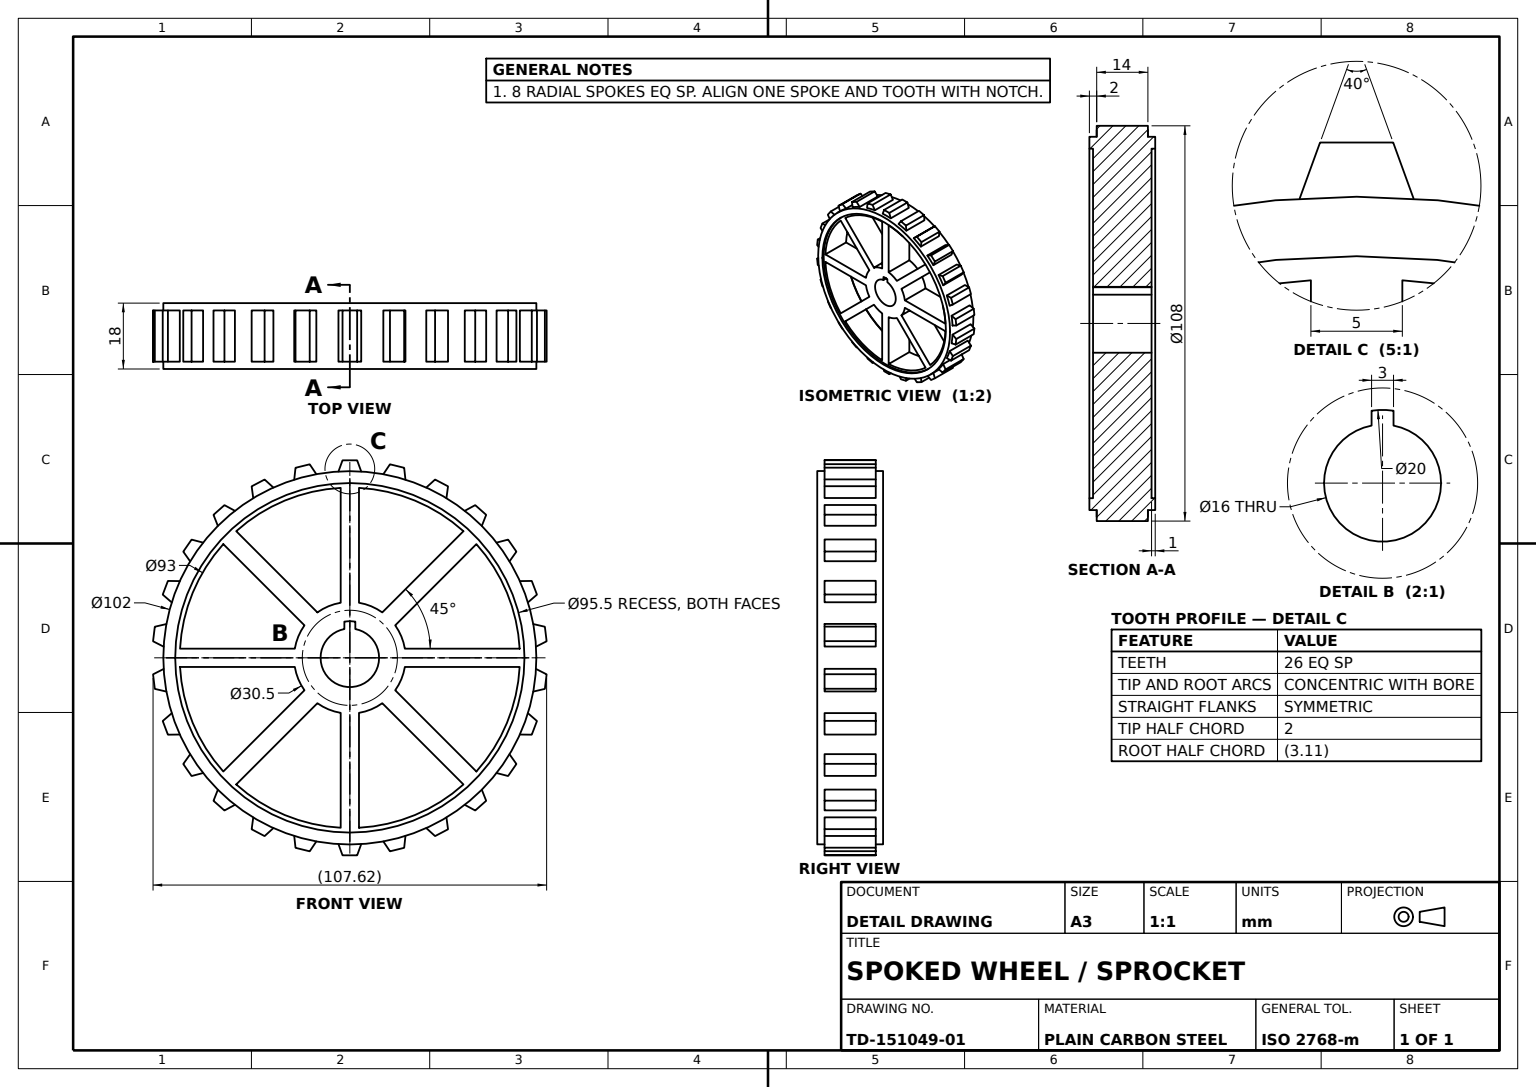
solid
v1 (51.165445,17.265493,7)
v2 (51.165445,17.265493,-7)
e1 v1 v2 LINE
v3 (48.700808,15.140385,7)
e2 v3 v1 LINE
v4 (48.700808,15.140385,-7)
e3 v3 v4 LINE
e4 v4 v2 LINE
face PLANE(AX(P(51.165445,17.265493,7),D(-0.653013985,0.757345849,0),D(-0.757345849,-0.653013985,0))) rev [-e1 -e2 e3 e4]
v5 (26.848745,46.852373,-7)
v6 (23.306921,48.711266,-7)
e5 v5 v6 CIRCLE(AX(P(0,0,-7),D(0,0,1),D(1,0,0)),54)
v7 (23.306921,48.711266,7)
e6 v7 v6 LINE
v8 (26.848745,46.852373,7)
e7 v8 v7 CIRCLE(AX(P(0,0,7),D(0,0,1),D(1,0,0)),54)
e8 v8 v5 LINE
face CYL(AX(P(0,0,7),D(0,0,-1),D(-1,0,0)),54) [e5 -e6 -e7 e8]
v9 (-34.287034,-41.718094,7)
v10 (-31.426051,-40.167192,7)
e9 v9 v10 LINE
v11 (-36.086337,-36.038539,7)
e10 v11 v10 CIRCLE(AX(P(0,0,7),D(0,0,1),D(1,0,0)),51)
v12 (-37.281077,-39.065603,7)
e11 v11 v12 LINE
e12 v12 v9 CIRCLE(AX(P(0,0,7),D(0,0,1),D(1,0,0)),54)
face PLANE(AX(P(0,0,7),D(0,0,1),D(1,0,0))) [e9 -e10 e11 e12]
v13 (53.810573,-4.519097,7)
v14 (50.908983,-3.045567,7)
e13 v13 v14 LINE
v15 (53.810573,-4.519097,-7)
e14 v13 v15 LINE
v16 (50.908983,-3.045567,-7)
e15 v15 v16 LINE
e16 v14 v16 LINE
face PLANE(AX(P(53.810573,-4.519097,7),D(-0.45279386,-0.891615231,0),D(0.891615231,-0.45279386,0))) rev [-e13 e14 e15 -e16]
v17 (-31.065143,34.600677,8)
v18 (-31.065143,34.600677,-8)
e17 v17 v18 LINE
v19 (-2.5,46.432747,-8)
e18 v18 v19 CIRCLE(AX(P(0,0,-8),D(0,0,-1),D(-1,0,0)),46.5)
v20 (-2.5,46.432747,8)
e19 v20 v19 LINE
e20 v20 v17 CIRCLE(AX(P(0,0,8),D(0,0,1),D(1,0,0)),46.5)
face CYL(AX(P(0,0,9),D(0,0,-1),D(-1,0,0)),46.5) rev [e17 e18 -e19 e20]
v21 (31.065143,34.600677,8)
v22 (2.5,46.432747,8)
e21 v21 v22 CIRCLE(AX(P(0,0,8),D(0,0,1),D(1,0,0)),46.5)
v23 (2.5,46.432747,-8)
e22 v22 v23 LINE
v24 (31.065143,34.600677,-8)
e23 v23 v24 CIRCLE(AX(P(0,0,-8),D(0,0,-1),D(-1,0,0)),46.5)
e24 v21 v24 LINE
face CYL(AX(P(0,0,9),D(0,0,-1),D(-1,0,0)),46.5) rev [e21 e22 e23 -e24]
v25 (51.165445,-17.265493,7)
v26 (48.700808,-15.140385,7)
e25 v25 v26 LINE
v27 (51.165445,-17.265493,-7)
e26 v25 v27 LINE
v28 (48.700808,-15.140385,-7)
e27 v27 v28 LINE
e28 v26 v28 LINE
face PLANE(AX(P(51.165445,-17.265493,7),D(-0.653013985,-0.757345849,0),D(0.757345849,-0.653013985,0))) rev [-e25 e26 e27 -e28]
v29 (-3.113039,-50.904901,-7)
v30 (-2,-53.96295,-7)
e29 v29 v30 LINE
v31 (-2,-53.96295,7)
e30 v31 v30 LINE
v32 (-3.113039,-50.904901,7)
e31 v32 v31 LINE
e32 v32 v29 LINE
face PLANE(AX(P(-2,-53.96295,7),D(0.939692621,0.342020143,0),D(-0.342020143,0.939692621,0))) rev [e29 -e30 -e31 e32]
v33 (-26.848745,-46.852373,7)
v34 (-26.848745,-46.852373,-7)
e33 v33 v34 LINE
v35 (-26.413146,-43.62735,7)
e34 v35 v33 LINE
v36 (-26.413146,-43.62735,-7)
e35 v35 v36 LINE
e36 v36 v34 LINE
face PLANE(AX(P(-26.848745,-46.852373,7),D(0.991001179,-0.133853139,0),D(0.133853139,0.991001179,0))) rev [-e33 -e34 e35 e36]
v37 (46.493011,20.961869,7)
e37 v3 v37 CIRCLE(AX(P(0,0,7),D(0,0,1),D(1,0,0)),51)
v38 (49.747025,21.005558,7)
e38 v1 v38 CIRCLE(AX(P(0,0,7),D(0,0,1),D(1,0,0)),54)
e39 v38 v37 LINE
face PLANE(AX(P(0,0,7),D(0,0,1),D(1,0,0))) [-e37 e2 e38 e39]
v39 (-20.900228,46.520753,-7)
v40 (-23.306921,48.711266,-7)
e40 v39 v40 LINE
v41 (-26.413146,43.62735,-7)
e41 v39 v41 CIRCLE(AX(P(0,0,-7),D(0,0,1),D(1,0,0)),51)
v42 (-26.848745,46.852373,-7)
e42 v42 v41 LINE
e43 v40 v42 CIRCLE(AX(P(0,0,-7),D(0,0,1),D(1,0,0)),54)
face PLANE(AX(P(0,0,-7),D(0,0,1),D(1,0,0))) rev [-e40 e41 -e42 -e43]
v43 (8.869726,12.40526,8)
e44 v43 v21 LINE
v44 (2.5,15.043686,8)
e45 v44 v43 CIRCLE(AX(P(0,0,8),D(0,0,-1),D(1,0,0)),15.25)
e46 v22 v44 LINE
v45 (-34.600677,31.065143,8)
v46 (-46.432747,2.5,8)
e47 v45 v46 CIRCLE(AX(P(0,0,8),D(0,0,1),D(1,0,0)),46.5)
v47 (-12.40526,8.869726,8)
e48 v47 v45 LINE
v48 (-15.043686,2.5,8)
e49 v48 v47 CIRCLE(AX(P(0,0,8),D(0,0,-1),D(1,0,0)),15.25)
e50 v46 v48 LINE
v49 (-8.869726,-12.40526,8)
v50 (-31.065143,-34.600677,8)
e51 v49 v50 LINE
v51 (-2.5,-15.043686,8)
e52 v51 v49 CIRCLE(AX(P(0,0,8),D(0,0,-1),D(1,0,0)),15.25)
v52 (-2.5,-46.432747,8)
e53 v52 v51 LINE
e54 v50 v52 CIRCLE(AX(P(0,0,8),D(0,0,1),D(1,0,0)),46.5)
v53 (-2.5,15.043686,8)
e55 v53 v20 LINE
v54 (-8.869726,12.40526,8)
e56 v54 v53 CIRCLE(AX(P(0,0,8),D(0,0,-1),D(1,0,0)),15.25)
e57 v17 v54 LINE
v55 (2.5,-15.043686,8)
v56 (2.5,-46.432747,8)
e58 v55 v56 LINE
v57 (8.869726,-12.40526,8)
e59 v57 v55 CIRCLE(AX(P(0,0,8),D(0,0,-1),D(1,0,0)),15.25)
v58 (31.065143,-34.600677,8)
e60 v58 v57 LINE
e61 v56 v58 CIRCLE(AX(P(0,0,8),D(0,0,1),D(1,0,0)),46.5)
v59 (-34.600677,-31.065143,8)
v60 (-12.40526,-8.869726,8)
e62 v59 v60 LINE
v61 (-46.432747,-2.5,8)
e63 v61 v59 CIRCLE(AX(P(0,0,8),D(0,0,1),D(1,0,0)),46.5)
v62 (-15.043686,-2.5,8)
e64 v62 v61 LINE
e65 v60 v62 CIRCLE(AX(P(0,0,8),D(0,0,-1),D(1,0,0)),15.25)
v63 (-47.75,0,8)
v64 (47.75,0,8)
e66 v63 v64 CIRCLE(AX(P(0,0,8),D(0,0,1),D(1,0,0)),47.75)
e67 v64 v63 CIRCLE(AX(P(0,0,8),D(0,0,1),D(1,0,0)),47.75)
v65 (1.5,9.88686,8)
v66 (1.5,7.858117,8)
e68 v65 v66 LINE
v67 (8,0,8)
e69 v67 v66 CIRCLE(AX(P(0,0,8),D(0,0,1),D(1,0,0)),8)
v68 (-8,0,8)
e70 v68 v67 CIRCLE(AX(P(0,0,8),D(0,0,1),D(1,0,0)),8)
v69 (-1.5,7.858117,8)
e71 v69 v68 CIRCLE(AX(P(0,0,8),D(0,0,1),D(1,0,0)),8)
v70 (-1.5,9.88686,8)
e72 v69 v70 LINE
e73 v70 v65 CIRCLE(AX(P(0,0,8),D(0,0,-1),D(1,0,0)),10)
v71 (15.043686,-2.5,8)
v72 (12.40526,-8.869726,8)
e74 v71 v72 CIRCLE(AX(P(0,0,8),D(0,0,-1),D(1,0,0)),15.25)
v73 (46.432747,-2.5,8)
e75 v73 v71 LINE
v74 (34.600677,-31.065143,8)
e76 v74 v73 CIRCLE(AX(P(0,0,8),D(0,0,1),D(1,0,0)),46.5)
e77 v72 v74 LINE
v75 (15.043686,2.5,8)
v76 (46.432747,2.5,8)
e78 v75 v76 LINE
v77 (12.40526,8.869726,8)
e79 v77 v75 CIRCLE(AX(P(0,0,8),D(0,0,-1),D(1,0,0)),15.25)
v78 (34.600677,31.065143,8)
e80 v78 v77 LINE
e81 v76 v78 CIRCLE(AX(P(0,0,8),D(0,0,1),D(1,0,0)),46.5)
face PLANE(AX(P(0,0,8),D(0,0,1),D(1,0,0))) [-e44 -e45 -e46 -e21] [-e47 -e48 -e49 -e50] [-e51 -e52 -e53 -e54] [-e20 -e55 -e56 -e57] [-e58 -e59 -e60 -e61] [-e62 -e63 -e64 -e65] [e66 e67] [e68 -e69 -e70 -e71 e72 e73] [-e74 -e75 -e76 -e77] [-e78 -e79 -e80 -e81]
v79 (9.159761,-50.170696,-7)
v80 (10.972296,-52.873516,-7)
e82 v79 v80 LINE
v81 (10.972296,-52.873516,7)
e83 v81 v80 LINE
v82 (9.159761,-50.170696,7)
e84 v82 v81 LINE
e85 v82 v79 LINE
face PLANE(AX(P(10.972296,-52.873516,7),D(0.830536083,0.556964823,0),D(-0.556964823,0.830536083,0))) rev [e82 -e83 -e84 e85]
v83 (15.043686,-2.5,-8)
e86 v71 v83 LINE
v84 (46.432747,-2.5,-8)
e87 v83 v84 LINE
e88 v73 v84 LINE
face PLANE(AX(P(46.432747,-2.5,9),D(0,-1,0),D(1,0,0))) [e86 e87 -e88 e75]
v85 (-34.600677,31.065143,-8)
e89 v45 v85 LINE
v86 (-12.40526,8.869726,-8)
e90 v85 v86 LINE
e91 v47 v86 LINE
face PLANE(AX(P(-12.40526,8.869726,9),D(-0.707106781,-0.707106781,0),D(0.707106781,-0.707106781,0))) [e89 e90 -e91 e48]
v87 (-48.700808,-15.140385,-7)
v88 (-51.165445,-17.265493,-7)
e92 v87 v88 LINE
v89 (-51.165445,-17.265493,7)
e93 v89 v88 LINE
v90 (-48.700808,-15.140385,7)
e94 v90 v89 LINE
e95 v90 v87 LINE
face PLANE(AX(P(-51.165445,-17.265493,7),D(0.653013985,-0.757345849,0),D(0.757345849,0.653013985,0))) rev [e92 -e93 -e94 e95]
v91 (50.158512,-9.226249,7)
v92 (53.328426,-8.489933,7)
e96 v91 v92 LINE
v93 (50.158512,-9.226249,-7)
e97 v91 v93 LINE
v94 (53.328426,-8.489933,-7)
e98 v93 v94 LINE
e99 v92 v94 LINE
face PLANE(AX(P(53.328426,-8.489933,7),D(-0.226259002,0.974067176,0),D(-0.974067176,-0.226259002,0))) rev [-e96 e97 e98 -e99]
v95 (14.856063,51.916254,-7)
v96 (10.972296,52.873516,-7)
e100 v95 v96 CIRCLE(AX(P(0,0,-7),D(0,0,1),D(1,0,0)),54)
v97 (10.972296,52.873516,7)
e101 v97 v96 LINE
v98 (14.856063,51.916254,7)
e102 v98 v97 CIRCLE(AX(P(0,0,7),D(0,0,1),D(1,0,0)),54)
e103 v98 v95 LINE
face CYL(AX(P(0,0,7),D(0,0,-1),D(-1,0,0)),54) [e100 -e101 -e102 e103]
v99 (34.287034,-41.718094,7)
v100 (34.287034,-41.718094,-7)
e104 v99 v100 LINE
v101 (37.281077,-39.065603,-7)
e105 v100 v101 CIRCLE(AX(P(0,0,-7),D(0,0,1),D(1,0,0)),54)
v102 (37.281077,-39.065603,7)
e106 v102 v101 LINE
e107 v99 v102 CIRCLE(AX(P(0,0,7),D(0,0,1),D(1,0,0)),54)
face CYL(AX(P(0,0,7),D(0,0,-1),D(-1,0,0)),54) [e104 e105 -e106 -e107]
v103 (-53.328426,8.489933,-7)
v104 (-53.810573,4.519097,-7)
e108 v103 v104 CIRCLE(AX(P(0,0,-7),D(0,0,1),D(1,0,0)),54)
v105 (-53.810573,4.519097,7)
e109 v105 v104 LINE
v106 (-53.328426,8.489933,7)
e110 v106 v105 CIRCLE(AX(P(0,0,7),D(0,0,1),D(1,0,0)),54)
e111 v106 v103 LINE
face CYL(AX(P(0,0,7),D(0,0,-1),D(-1,0,0)),54) [e108 -e109 -e110 e111]
v107 (20.900228,-46.520753,-7)
v108 (23.306921,-48.711266,-7)
e112 v107 v108 LINE
v109 (23.306921,-48.711266,7)
e113 v109 v108 LINE
v110 (20.900228,-46.520753,7)
e114 v110 v109 LINE
e115 v110 v107 LINE
face PLANE(AX(P(23.306921,-48.711266,7),D(0.673111807,0.739540732,0),D(-0.739540732,0.673111807,0))) rev [e112 -e113 -e114 e115]
v111 (50.908983,3.045567,7)
v112 (50.908983,3.045567,-7)
e116 v111 v112 LINE
v113 (53.810573,4.519097,-7)
e117 v112 v113 LINE
v114 (53.810573,4.519097,7)
e118 v114 v113 LINE
e119 v111 v114 LINE
face PLANE(AX(P(53.810573,4.519097,7),D(-0.45279386,0.891615231,0),D(-0.891615231,-0.45279386,0))) rev [e116 e117 -e118 -e119]
v115 (-37.281077,39.065603,7)
v116 (-36.086337,36.038539,7)
e120 v115 v116 LINE
v117 (-37.281077,39.065603,-7)
e121 v115 v117 LINE
v118 (-36.086337,36.038539,-7)
e122 v117 v118 LINE
e123 v116 v118 LINE
face PLANE(AX(P(-37.281077,39.065603,7),D(0.930171333,0.367125715,0),D(-0.367125715,0.930171333,0))) rev [-e120 e121 e122 -e123]
v119 (-46.432747,-2.5,-8)
e124 v61 v119 LINE
v120 (-15.043686,-2.5,-8)
e125 v119 v120 LINE
e126 v62 v120 LINE
face PLANE(AX(P(-15.043686,-2.5,9),D(0,-1,0),D(1,0,0))) [e124 e125 -e126 e64]
v121 (31.426051,40.167192,7)
v122 (31.426051,40.167192,-7)
e127 v121 v122 LINE
v123 (34.287034,41.718094,7)
e128 v123 v121 LINE
v124 (34.287034,41.718094,-7)
e129 v123 v124 LINE
e130 v124 v122 LINE
face PLANE(AX(P(34.287034,41.718094,7),D(0.47656872,-0.879137222,0),D(0.879137222,0.47656872,0))) rev [-e127 -e128 e129 e130]
v125 (-34.287034,41.718094,7)
e131 v125 v115 CIRCLE(AX(P(0,0,7),D(0,0,1),D(1,0,0)),54)
v126 (-31.426051,40.167192,7)
e132 v126 v116 CIRCLE(AX(P(0,0,7),D(0,0,1),D(1,0,0)),51)
e133 v126 v125 LINE
face PLANE(AX(P(0,0,7),D(0,0,1),D(1,0,0))) [e131 e120 -e132 e133]
v127 (-15.043686,2.5,-8)
v128 (-46.432747,2.5,-8)
e134 v127 v128 LINE
e135 v46 v128 LINE
e136 v48 v127 LINE
face PLANE(AX(P(-46.432747,2.5,9),D(0,1,0),D(-1,0,0))) [e134 -e135 e50 e136]
v129 (-36.086337,-36.038539,-7)
v130 (-31.426051,-40.167192,-7)
e137 v129 v130 CIRCLE(AX(P(0,0,-7),D(0,0,1),D(1,0,0)),51)
v131 (-34.287034,-41.718094,-7)
e138 v131 v130 LINE
v132 (-37.281077,-39.065603,-7)
e139 v132 v131 CIRCLE(AX(P(0,0,-7),D(0,0,1),D(1,0,0)),54)
e140 v129 v132 LINE
face PLANE(AX(P(0,0,-7),D(0,0,1),D(1,0,0))) rev [e137 -e138 -e139 -e140]
v133 (-49.747025,-21.005558,7)
v134 (-49.747025,-21.005558,-7)
e141 v133 v134 LINE
v135 (-46.493011,-20.961869,-7)
e142 v134 v135 LINE
v136 (-46.493011,-20.961869,7)
e143 v136 v135 LINE
e144 v133 v136 LINE
face PLANE(AX(P(-49.747025,-21.005558,7),D(-0.013425206,0.999909878,0),D(-0.999909878,-0.013425206,0))) rev [e141 e142 -e143 -e144]
v137 (-14.856063,51.916254,-7)
v138 (-15.20492,48.680699,-7)
e145 v137 v138 LINE
v139 (-10.972296,52.873516,-7)
e146 v139 v137 CIRCLE(AX(P(0,0,-7),D(0,0,1),D(1,0,0)),54)
v140 (-9.159761,50.170696,-7)
e147 v140 v139 LINE
e148 v140 v138 CIRCLE(AX(P(0,0,-7),D(0,0,1),D(1,0,0)),51)
face PLANE(AX(P(0,0,-7),D(0,0,1),D(1,0,0))) rev [-e145 -e146 -e147 e148]
e149 v89 v133 CIRCLE(AX(P(0,0,7),D(0,0,1),D(1,0,0)),54)
e150 v90 v136 CIRCLE(AX(P(0,0,7),D(0,0,1),D(1,0,0)),51)
face PLANE(AX(P(0,0,7),D(0,0,1),D(1,0,0))) [e94 e149 e144 -e150]
v141 (-49.747025,21.005558,-7)
v142 (-51.165445,17.265493,-7)
e151 v141 v142 CIRCLE(AX(P(0,0,-7),D(0,0,1),D(1,0,0)),54)
v143 (-51.165445,17.265493,7)
e152 v143 v142 LINE
v144 (-49.747025,21.005558,7)
e153 v144 v143 CIRCLE(AX(P(0,0,7),D(0,0,1),D(1,0,0)),54)
e154 v144 v141 LINE
face CYL(AX(P(0,0,7),D(0,0,-1),D(-1,0,0)),54) [e151 -e152 -e153 e154]
v145 (15.20492,-48.680699,7)
v146 (15.20492,-48.680699,-7)
e155 v145 v146 LINE
v147 (14.856063,-51.916254,7)
e156 v147 v145 LINE
v148 (14.856063,-51.916254,-7)
e157 v147 v148 LINE
e158 v148 v146 LINE
face PLANE(AX(P(14.856063,-51.916254,7),D(-0.994237639,0.107198496,0),D(-0.107198496,-0.994237639,0))) rev [-e155 -e156 e157 e158]
v149 (15.043686,2.5,-8)
e159 v75 v149 LINE
v150 (12.40526,8.869726,-8)
e160 v149 v150 CIRCLE(AX(P(0,0,-8),D(0,0,1),D(-1,0,0)),15.25)
e161 v77 v150 LINE
face CYL(AX(P(0,0,9),D(0,0,-1),D(-1,0,0)),15.25) [e159 e160 -e161 e79]
v151 (43.274508,32.300417,-7)
v152 (40.125505,31.479261,-7)
e162 v151 v152 LINE
v153 (40.125505,31.479261,7)
e163 v153 v152 LINE
v154 (43.274508,32.300417,7)
e164 v154 v153 LINE
e165 v154 v151 LINE
face PLANE(AX(P(43.274508,32.300417,7),D(0.252329191,-0.967641452,0),D(0.967641452,0.252329191,0))) rev [e162 -e163 -e164 e165]
v155 (-2.5,-46.432747,-8)
v156 (-31.065143,-34.600677,-8)
e166 v155 v156 CIRCLE(AX(P(0,0,-8),D(0,0,-1),D(-1,0,0)),46.5)
e167 v50 v156 LINE
e168 v52 v155 LINE
face CYL(AX(P(0,0,9),D(0,0,-1),D(-1,0,0)),46.5) rev [e166 -e167 e54 e168]
e169 v128 v85 CIRCLE(AX(P(0,0,-8),D(0,0,-1),D(-1,0,0)),46.5)
face CYL(AX(P(0,0,9),D(0,0,-1),D(-1,0,0)),46.5) rev [e169 -e89 e47 e135]
v157 (26.413146,43.62735,7)
e170 v157 v8 LINE
v158 (26.413146,43.62735,-7)
e171 v157 v158 LINE
e172 v158 v5 LINE
face PLANE(AX(P(26.848745,46.852373,7),D(-0.991001179,0.133853139,0),D(-0.133853139,-0.991001179,0))) rev [-e170 e171 e172 -e8]
v159 (-8.869726,-12.40526,-8)
e173 v156 v159 LINE
e174 v49 v159 LINE
face PLANE(AX(P(-8.869726,-12.40526,9),D(0.707106781,-0.707106781,0),D(0.707106781,0.707106781,0))) [e167 e173 -e174 e51]
v160 (46.432747,2.5,-8)
e175 v76 v160 LINE
e176 v160 v149 LINE
face PLANE(AX(P(15.043686,2.5,9),D(0,1,0),D(-1,0,0))) [-e159 e78 e175 e176]
v161 (2,53.96295,-7)
v162 (-2,53.96295,-7)
e177 v161 v162 CIRCLE(AX(P(0,0,-7),D(0,0,1),D(1,0,0)),54)
v163 (-2,53.96295,7)
e178 v163 v162 LINE
v164 (2,53.96295,7)
e179 v164 v163 CIRCLE(AX(P(0,0,7),D(0,0,1),D(1,0,0)),54)
e180 v164 v161 LINE
face CYL(AX(P(0,0,7),D(0,0,-1),D(-1,0,0)),54) [e177 -e178 -e179 e180]
v165 (31.065143,-34.600677,-8)
v166 (2.5,-46.432747,-8)
e181 v165 v166 CIRCLE(AX(P(0,0,-8),D(0,0,-1),D(-1,0,0)),46.5)
e182 v56 v166 LINE
e183 v58 v165 LINE
face CYL(AX(P(0,0,9),D(0,0,-1),D(-1,0,0)),46.5) rev [e181 -e182 e61 e183]
v167 (46.493011,20.961869,-7)
e184 v37 v167 LINE
v168 (49.747025,21.005558,-7)
e185 v38 v168 LINE
e186 v168 v167 LINE
face PLANE(AX(P(49.747025,21.005558,7),D(0.013425206,-0.999909878,0),D(0.999909878,0.013425206,0))) rev [-e184 -e39 e185 e186]
v169 (-34.287034,41.718094,-7)
e187 v125 v169 LINE
e188 v169 v117 CIRCLE(AX(P(0,0,-7),D(0,0,1),D(1,0,0)),54)
face CYL(AX(P(0,0,7),D(0,0,-1),D(-1,0,0)),54) [-e121 -e131 e187 e188]
e189 v92 v13 CIRCLE(AX(P(0,0,7),D(0,0,1),D(1,0,0)),54)
e190 v91 v14 CIRCLE(AX(P(0,0,7),D(0,0,1),D(1,0,0)),51)
face PLANE(AX(P(0,0,7),D(0,0,1),D(1,0,0))) [e96 e189 e13 -e190]
v170 (-40.125505,31.479261,7)
v171 (-43.274508,32.300417,7)
e191 v170 v171 LINE
v172 (-40.125505,31.479261,-7)
e192 v170 v172 LINE
v173 (-43.274508,32.300417,-7)
e193 v172 v173 LINE
e194 v171 v173 LINE
face PLANE(AX(P(-43.274508,32.300417,7),D(-0.252329191,-0.967641452,0),D(0.967641452,-0.252329191,0))) rev [-e191 e192 e193 -e194]
v174 (-12.40526,-8.869726,-8)
e195 v60 v174 LINE
v175 (-34.600677,-31.065143,-8)
e196 v174 v175 LINE
e197 v59 v175 LINE
face PLANE(AX(P(-34.600677,-31.065143,9),D(-0.707106781,0.707106781,0),D(-0.707106781,-0.707106781,0))) [e195 e196 -e197 e62]
v176 (49.747025,-21.005558,7)
e198 v176 v25 CIRCLE(AX(P(0,0,7),D(0,0,1),D(1,0,0)),54)
v177 (49.747025,-21.005558,-7)
e199 v176 v177 LINE
e200 v177 v27 CIRCLE(AX(P(0,0,-7),D(0,0,1),D(1,0,0)),54)
face CYL(AX(P(0,0,7),D(0,0,-1),D(-1,0,0)),54) [-e198 e199 e200 -e26]
v178 (-2.5,15.043686,-8)
e201 v53 v178 LINE
v179 (-8.869726,12.40526,-8)
e202 v178 v179 CIRCLE(AX(P(0,0,-8),D(0,0,1),D(-1,0,0)),15.25)
e203 v54 v179 LINE
face CYL(AX(P(0,0,9),D(0,0,-1),D(-1,0,0)),15.25) [e201 e202 -e203 e56]
v180 (-45.546767,29.008482,7)
v181 (-45.546767,29.008482,-7)
e204 v180 v181 LINE
e205 v171 v180 CIRCLE(AX(P(0,0,7),D(0,0,1),D(1,0,0)),54)
e206 v173 v181 CIRCLE(AX(P(0,0,-7),D(0,0,1),D(1,0,0)),54)
face CYL(AX(P(0,0,7),D(0,0,-1),D(-1,0,0)),54) [-e204 -e205 e194 e206]
v182 (-50.908983,3.045567,7)
v183 (-50.908983,3.045567,-7)
e207 v182 v183 LINE
e208 v105 v182 LINE
e209 v104 v183 LINE
face PLANE(AX(P(-53.810573,4.519097,7),D(0.45279386,0.891615231,0),D(-0.891615231,0.45279386,0))) rev [-e207 -e208 e109 e209]
v184 (-1.5,9.88686,-8)
e210 v184 v70 LINE
v185 (1.5,9.88686,-8)
e211 v185 v184 CIRCLE(AX(P(0,0,-8),D(0,0,1),D(-1,0,0)),10)
e212 v185 v65 LINE
face CYL(AX(P(0,0,-9),D(0,0,1),D(1,0,0)),10) rev [-e73 -e210 -e211 e212]
v186 (-14.856063,-51.916254,7)
v187 (-14.856063,-51.916254,-7)
e213 v186 v187 LINE
v188 (-15.20492,-48.680699,7)
e214 v188 v186 LINE
v189 (-15.20492,-48.680699,-7)
e215 v188 v189 LINE
e216 v189 v187 LINE
face PLANE(AX(P(-14.856063,-51.916254,7),D(0.994237639,0.107198496,0),D(-0.107198496,0.994237639,0))) rev [-e213 -e214 e215 e216]
v190 (8.869726,-12.40526,-8)
e217 v57 v190 LINE
e218 v190 v165 LINE
face PLANE(AX(P(31.065143,-34.600677,9),D(-0.707106781,-0.707106781,0),D(0.707106781,-0.707106781,0))) [e60 e217 e218 -e183]
v191 (45.546767,29.008482,7)
e219 v191 v154 CIRCLE(AX(P(0,0,7),D(0,0,1),D(1,0,0)),54)
v192 (43.66232,26.355299,7)
e220 v192 v153 CIRCLE(AX(P(0,0,7),D(0,0,1),D(1,0,0)),51)
e221 v192 v191 LINE
face PLANE(AX(P(0,0,7),D(0,0,1),D(1,0,0))) [e219 e164 -e220 e221]
v193 (45.546767,29.008482,-7)
e222 v193 v151 CIRCLE(AX(P(0,0,-7),D(0,0,1),D(1,0,0)),54)
v194 (43.66232,26.355299,-7)
e223 v194 v193 LINE
e224 v194 v152 CIRCLE(AX(P(0,0,-7),D(0,0,1),D(1,0,0)),51)
face PLANE(AX(P(0,0,-7),D(0,0,1),D(1,0,0))) rev [-e162 -e222 -e223 e224]
v195 (45.546767,-29.008482,-7)
v196 (43.66232,-26.355299,-7)
e225 v195 v196 LINE
v197 (43.66232,-26.355299,7)
e226 v197 v196 LINE
v198 (45.546767,-29.008482,7)
e227 v198 v197 LINE
e228 v198 v195 LINE
face PLANE(AX(P(45.546767,-29.008482,7),D(-0.81528331,-0.57906228,0),D(0.57906228,-0.81528331,0))) rev [e225 -e226 -e227 e228]
e229 v192 v194 LINE
e230 v191 v193 LINE
face PLANE(AX(P(45.546767,29.008482,7),D(-0.81528331,0.57906228,0),D(-0.57906228,-0.81528331,0))) rev [e229 e223 -e230 -e221]
v199 (31.426051,-40.167192,7)
e231 v199 v99 LINE
v200 (36.086337,-36.038539,7)
e232 v102 v200 LINE
e233 v199 v200 CIRCLE(AX(P(0,0,7),D(0,0,1),D(1,0,0)),51)
face PLANE(AX(P(0,0,7),D(0,0,1),D(1,0,0))) [e231 e107 e232 -e233]
v201 (-10.972296,-52.873516,-7)
v202 (-9.159761,-50.170696,-7)
e234 v201 v202 LINE
v203 (-9.159761,-50.170696,7)
e235 v203 v202 LINE
v204 (-10.972296,-52.873516,7)
e236 v204 v203 LINE
e237 v204 v201 LINE
face PLANE(AX(P(-10.972296,-52.873516,7),D(-0.830536083,0.556964823,0),D(-0.556964823,-0.830536083,0))) rev [e234 -e235 -e236 e237]
v205 (36.086337,36.038539,7)
v206 (37.281077,39.065603,7)
e238 v205 v206 LINE
e239 v206 v123 CIRCLE(AX(P(0,0,7),D(0,0,1),D(1,0,0)),54)
e240 v205 v121 CIRCLE(AX(P(0,0,7),D(0,0,1),D(1,0,0)),51)
face PLANE(AX(P(0,0,7),D(0,0,1),D(1,0,0))) [e238 e239 e128 -e240]
e241 v82 v145 CIRCLE(AX(P(0,0,7),D(0,0,1),D(1,0,0)),51)
e242 v81 v147 CIRCLE(AX(P(0,0,7),D(0,0,1),D(1,0,0)),54)
face PLANE(AX(P(0,0,7),D(0,0,1),D(1,0,0))) [-e241 e84 e242 e156]
v207 (34.600677,31.065143,-8)
e243 v207 v160 CIRCLE(AX(P(0,0,-8),D(0,0,-1),D(-1,0,0)),46.5)
e244 v78 v207 LINE
face CYL(AX(P(0,0,9),D(0,0,-1),D(-1,0,0)),46.5) rev [e243 -e175 e81 e244]
v208 (-46.493011,20.961869,7)
v209 (-46.493011,20.961869,-7)
e245 v208 v209 LINE
e246 v209 v141 LINE
e247 v208 v144 LINE
face PLANE(AX(P(-49.747025,21.005558,7),D(-0.013425206,-0.999909878,0),D(0.999909878,-0.013425206,0))) rev [e245 e246 -e154 -e247]
v210 (-26.848745,46.852373,7)
e248 v210 v42 LINE
v211 (-26.413146,43.62735,7)
e249 v211 v41 LINE
e250 v210 v211 LINE
face PLANE(AX(P(-26.848745,46.852373,7),D(0.991001179,0.133853139,0),D(-0.133853139,0.991001179,0))) rev [e248 e42 -e249 -e250]
v212 (-2.5,-15.043686,-8)
e251 v51 v212 LINE
e252 v212 v155 LINE
face PLANE(AX(P(-2.5,-46.432747,9),D(-1,0,0),D(0,-1,0))) [-e168 e53 e251 e252]
v213 (53.328426,8.489933,7)
e253 v114 v213 CIRCLE(AX(P(0,0,7),D(0,0,1),D(1,0,0)),54)
v214 (50.158512,9.226249,7)
e254 v213 v214 LINE
e255 v111 v214 CIRCLE(AX(P(0,0,7),D(0,0,1),D(1,0,0)),51)
face PLANE(AX(P(0,0,7),D(0,0,1),D(1,0,0))) [e253 e254 -e255 e119]
e256 v80 v148 CIRCLE(AX(P(0,0,-7),D(0,0,1),D(1,0,0)),54)
e257 v79 v146 CIRCLE(AX(P(0,0,-7),D(0,0,1),D(1,0,0)),51)
face PLANE(AX(P(0,0,-7),D(0,0,1),D(1,0,0))) rev [-e158 -e256 -e82 e257]
e258 v189 v202 CIRCLE(AX(P(0,0,-7),D(0,0,1),D(1,0,0)),51)
e259 v187 v201 CIRCLE(AX(P(0,0,-7),D(0,0,1),D(1,0,0)),54)
face PLANE(AX(P(0,0,-7),D(0,0,1),D(1,0,0))) rev [-e216 e258 -e234 -e259]
v215 (-51,0,9)
v216 (-51,0,-9)
e260 v215 v216 LINE
v217 (51,0,9)
e261 v217 v215 CIRCLE(AX(P(0,0,9),D(0,0,1),D(1,0,0)),51)
v218 (51,0,-9)
e262 v217 v218 LINE
e263 v218 v216 CIRCLE(AX(P(0,0,-9),D(0,0,1),D(1,0,0)),51)
v219 (-20.900228,46.520753,7)
e264 v219 v39 LINE
e265 v219 v211 CIRCLE(AX(P(0,0,7),D(0,0,1),D(1,0,0)),51)
e266 v4 v167 CIRCLE(AX(P(0,0,-7),D(0,0,1),D(1,0,0)),51)
v220 (20.900228,46.520753,7)
e267 v157 v220 CIRCLE(AX(P(0,0,7),D(0,0,1),D(1,0,0)),51)
v221 (20.900228,46.520753,-7)
e268 v220 v221 LINE
e269 v158 v221 CIRCLE(AX(P(0,0,-7),D(0,0,1),D(1,0,0)),51)
v222 (36.086337,36.038539,-7)
e270 v205 v222 LINE
e271 v222 v122 CIRCLE(AX(P(0,0,-7),D(0,0,1),D(1,0,0)),51)
v223 (-50.158512,9.226249,-7)
e272 v223 v183 CIRCLE(AX(P(0,0,-7),D(0,0,1),D(1,0,0)),51)
v224 (-50.158512,9.226249,7)
e273 v224 v223 LINE
e274 v224 v182 CIRCLE(AX(P(0,0,7),D(0,0,1),D(1,0,0)),51)
v225 (3.113039,50.904901,7)
v226 (-3.113039,50.904901,7)
e275 v225 v226 CIRCLE(AX(P(0,0,7),D(0,0,1),D(1,0,0)),51)
v227 (-3.113039,50.904901,-7)
e276 v226 v227 LINE
v228 (3.113039,50.904901,-7)
e277 v228 v227 CIRCLE(AX(P(0,0,-7),D(0,0,1),D(1,0,0)),51)
e278 v225 v228 LINE
v229 (-43.66232,26.355299,7)
e279 v170 v229 CIRCLE(AX(P(0,0,7),D(0,0,1),D(1,0,0)),51)
v230 (-43.66232,26.355299,-7)
e280 v229 v230 LINE
e281 v172 v230 CIRCLE(AX(P(0,0,-7),D(0,0,1),D(1,0,0)),51)
v231 (-9.159761,50.170696,7)
e282 v231 v140 LINE
v232 (-15.20492,48.680699,7)
e283 v231 v232 CIRCLE(AX(P(0,0,7),D(0,0,1),D(1,0,0)),51)
e284 v232 v138 LINE
v233 (-48.700808,15.140385,7)
v234 (-48.700808,15.140385,-7)
e285 v233 v234 LINE
e286 v209 v234 CIRCLE(AX(P(0,0,-7),D(0,0,1),D(1,0,0)),51)
e287 v208 v233 CIRCLE(AX(P(0,0,7),D(0,0,1),D(1,0,0)),51)
v235 (50.158512,9.226249,-7)
e288 v214 v235 LINE
e289 v112 v235 CIRCLE(AX(P(0,0,-7),D(0,0,1),D(1,0,0)),51)
v236 (15.20492,48.680699,7)
v237 (9.159761,50.170696,7)
e290 v236 v237 CIRCLE(AX(P(0,0,7),D(0,0,1),D(1,0,0)),51)
v238 (9.159761,50.170696,-7)
e291 v237 v238 LINE
v239 (15.20492,48.680699,-7)
e292 v239 v238 CIRCLE(AX(P(0,0,-7),D(0,0,1),D(1,0,0)),51)
e293 v236 v239 LINE
v240 (-31.426051,40.167192,-7)
e294 v126 v240 LINE
e295 v240 v118 CIRCLE(AX(P(0,0,-7),D(0,0,1),D(1,0,0)),51)
face CYL(AX(P(0,0,9),D(0,0,-1),D(-1,0,0)),51) [-e260 -e261 e262 e263] [-e41 -e264 e265 e249] [-e3 e37 e184 -e266] [-e171 e267 e268 -e269] [-e229 e220 e163 -e224] [-e270 e240 e127 -e271] [-e272 -e273 e274 e207] [e275 e276 -e277 -e278] [e279 e280 -e281 -e192] [-e282 e283 e284 -e148] [e285 -e286 -e245 e287] [-e116 e255 e288 -e289] [e290 e291 -e292 -e293] [-e294 e132 e123 -e295]
v241 (34.600677,-31.065143,-8)
e296 v84 v241 CIRCLE(AX(P(0,0,-8),D(0,0,-1),D(-1,0,0)),46.5)
e297 v74 v241 LINE
face CYL(AX(P(0,0,9),D(0,0,-1),D(-1,0,0)),46.5) rev [e76 e88 e296 -e297]
v242 (8,0,-8)
e298 v67 v242 LINE
v243 (-8,0,-8)
e299 v242 v243 CIRCLE(AX(P(0,0,-8),D(0,0,-1),D(-1,0,0)),8)
e300 v68 v243 LINE
face CYL(AX(P(0,0,9),D(0,0,-1),D(-1,0,0)),8) rev [e298 e299 -e300 e70]
v244 (-23.306921,-48.711266,7)
v245 (-20.900228,-46.520753,7)
e301 v244 v245 LINE
e302 v35 v245 CIRCLE(AX(P(0,0,7),D(0,0,1),D(1,0,0)),51)
e303 v33 v244 CIRCLE(AX(P(0,0,7),D(0,0,1),D(1,0,0)),54)
face PLANE(AX(P(0,0,7),D(0,0,1),D(1,0,0))) [e301 -e302 e34 e303]
v246 (53.328426,8.489933,-7)
e304 v213 v246 LINE
e305 v113 v246 CIRCLE(AX(P(0,0,-7),D(0,0,1),D(1,0,0)),54)
face CYL(AX(P(0,0,7),D(0,0,-1),D(-1,0,0)),54) [-e304 -e253 e118 e305]
e306 v7 v220 LINE
e307 v6 v221 LINE
face PLANE(AX(P(23.306921,48.711266,7),D(0.673111807,-0.739540732,0),D(0.739540732,0.673111807,0))) rev [-e306 e6 e307 -e268]
e308 v9 v131 LINE
e309 v10 v130 LINE
face PLANE(AX(P(-34.287034,-41.718094,7),D(-0.47656872,0.879137222,0),D(-0.879137222,-0.47656872,0))) rev [-e9 e308 e138 -e309]
e310 v96 v238 LINE
e311 v97 v237 LINE
face PLANE(AX(P(10.972296,52.873516,7),D(0.830536083,-0.556964823,0),D(0.556964823,0.830536083,0))) rev [e101 e310 -e291 -e311]
v247 (-45.546767,-29.008482,7)
v248 (-43.274508,-32.300417,7)
e312 v247 v248 CIRCLE(AX(P(0,0,7),D(0,0,1),D(1,0,0)),54)
v249 (-40.125505,-31.479261,7)
e313 v248 v249 LINE
v250 (-43.66232,-26.355299,7)
e314 v250 v249 CIRCLE(AX(P(0,0,7),D(0,0,1),D(1,0,0)),51)
e315 v250 v247 LINE
face PLANE(AX(P(0,0,7),D(0,0,1),D(1,0,0))) [e312 e313 -e314 e315]
e316 v225 v164 LINE
e317 v163 v226 LINE
face PLANE(AX(P(0,0,7),D(0,0,1),D(1,0,0))) [-e275 e316 e179 e317]
e318 v2 v168 CIRCLE(AX(P(0,0,-7),D(0,0,1),D(1,0,0)),54)
face PLANE(AX(P(0,0,-7),D(0,0,1),D(1,0,0))) rev [-e318 -e4 e266 -e186]
e319 v150 v207 LINE
face PLANE(AX(P(34.600677,31.065143,9),D(0.707106781,-0.707106781,0),D(0.707106781,0.707106781,0))) [e319 -e244 e80 e161]
e320 v179 v18 LINE
face PLANE(AX(P(-31.065143,34.600677,9),D(0.707106781,0.707106781,0),D(-0.707106781,0.707106781,0))) [e203 e320 -e17 e57]
e321 v236 v98 LINE
face PLANE(AX(P(0,0,7),D(0,0,1),D(1,0,0))) [e321 e102 e311 -e290]
v251 (-23.306921,48.711266,7)
e322 v219 v251 LINE
e323 v251 v210 CIRCLE(AX(P(0,0,7),D(0,0,1),D(1,0,0)),54)
face PLANE(AX(P(0,0,7),D(0,0,1),D(1,0,0))) [e322 e323 e250 -e265]
v252 (2.5,15.043686,-8)
e324 v252 v23 LINE
e325 v44 v252 LINE
face PLANE(AX(P(2.5,46.432747,9),D(1,0,0),D(0,1,0))) [e324 -e22 e46 e325]
v253 (8.869726,12.40526,-8)
e326 v24 v253 LINE
e327 v43 v253 LINE
face PLANE(AX(P(8.869726,12.40526,9),D(-0.707106781,0.707106781,0),D(-0.707106781,-0.707106781,0))) [e24 e326 -e327 e44]
e328 v216 v218 CIRCLE(AX(P(0,0,-9),D(0,0,1),D(1,0,0)),51)
e329 v215 v217 CIRCLE(AX(P(0,0,9),D(0,0,1),D(1,0,0)),51)
v254 (-50.908983,-3.045567,7)
v255 (-50.158512,-9.226249,7)
e330 v254 v255 CIRCLE(AX(P(0,0,7),D(0,0,1),D(1,0,0)),51)
v256 (-50.158512,-9.226249,-7)
e331 v255 v256 LINE
v257 (-50.908983,-3.045567,-7)
e332 v257 v256 CIRCLE(AX(P(0,0,-7),D(0,0,1),D(1,0,0)),51)
e333 v254 v257 LINE
e334 v93 v16 CIRCLE(AX(P(0,0,-7),D(0,0,1),D(1,0,0)),51)
v258 (-20.900228,-46.520753,-7)
e335 v36 v258 CIRCLE(AX(P(0,0,-7),D(0,0,1),D(1,0,0)),51)
e336 v245 v258 LINE
v259 (26.413146,-43.62735,7)
e337 v110 v259 CIRCLE(AX(P(0,0,7),D(0,0,1),D(1,0,0)),51)
v260 (26.413146,-43.62735,-7)
e338 v259 v260 LINE
e339 v107 v260 CIRCLE(AX(P(0,0,-7),D(0,0,1),D(1,0,0)),51)
v261 (36.086337,-36.038539,-7)
e340 v200 v261 LINE
v262 (31.426051,-40.167192,-7)
e341 v262 v261 CIRCLE(AX(P(0,0,-7),D(0,0,1),D(1,0,0)),51)
e342 v199 v262 LINE
v263 (3.113039,-50.904901,-7)
e343 v29 v263 CIRCLE(AX(P(0,0,-7),D(0,0,1),D(1,0,0)),51)
v264 (3.113039,-50.904901,7)
e344 v32 v264 CIRCLE(AX(P(0,0,7),D(0,0,1),D(1,0,0)),51)
e345 v264 v263 LINE
e346 v188 v203 CIRCLE(AX(P(0,0,7),D(0,0,1),D(1,0,0)),51)
e347 v11 v129 LINE
v265 (46.493011,-20.961869,-7)
e348 v265 v28 CIRCLE(AX(P(0,0,-7),D(0,0,1),D(1,0,0)),51)
v266 (46.493011,-20.961869,7)
e349 v266 v265 LINE
e350 v266 v26 CIRCLE(AX(P(0,0,7),D(0,0,1),D(1,0,0)),51)
v267 (-43.66232,-26.355299,-7)
e351 v250 v267 LINE
v268 (-40.125505,-31.479261,-7)
e352 v249 v268 LINE
e353 v267 v268 CIRCLE(AX(P(0,0,-7),D(0,0,1),D(1,0,0)),51)
v269 (40.125505,-31.479261,7)
v270 (40.125505,-31.479261,-7)
e354 v269 v270 LINE
e355 v269 v197 CIRCLE(AX(P(0,0,7),D(0,0,1),D(1,0,0)),51)
e356 v270 v196 CIRCLE(AX(P(0,0,-7),D(0,0,1),D(1,0,0)),51)
e357 v87 v135 CIRCLE(AX(P(0,0,-7),D(0,0,1),D(1,0,0)),51)
face CYL(AX(P(0,0,9),D(0,0,-1),D(-1,0,0)),51) [e328 -e262 -e329 e260] [e330 e331 -e332 -e333] [-e97 e190 e16 -e334] [-e335 -e35 e302 e336] [-e115 e337 e338 -e339] [e233 e340 -e341 -e342] [-e343 -e32 e344 e345] [e346 e235 -e258 -e215] [e10 e309 -e137 -e347] [e28 -e348 -e349 e350] [-e351 e314 e352 -e353] [-e85 e241 e155 -e257] [-e354 e355 e226 -e356] [-e357 -e95 e150 e143]
v271 (-23.306921,-48.711266,-7)
e358 v271 v258 LINE
e359 v34 v271 CIRCLE(AX(P(0,0,-7),D(0,0,1),D(1,0,0)),54)
face PLANE(AX(P(0,0,-7),D(0,0,1),D(1,0,0))) rev [-e36 e335 -e358 -e359]
v272 (26.848745,-46.852373,-7)
e360 v108 v272 CIRCLE(AX(P(0,0,-7),D(0,0,1),D(1,0,0)),54)
v273 (26.848745,-46.852373,7)
e361 v273 v272 LINE
e362 v109 v273 CIRCLE(AX(P(0,0,7),D(0,0,1),D(1,0,0)),54)
face CYL(AX(P(0,0,7),D(0,0,-1),D(-1,0,0)),54) [e113 e360 -e361 -e362]
e363 v246 v235 LINE
face PLANE(AX(P(53.328426,8.489933,7),D(-0.226259002,-0.974067176,0),D(0.974067176,-0.226259002,0))) rev [e304 e363 -e288 -e254]
e364 v224 v106 LINE
face PLANE(AX(P(0,0,7),D(0,0,1),D(1,0,0))) [e110 e208 -e274 e364]
e365 v120 v174 CIRCLE(AX(P(0,0,-8),D(0,0,1),D(-1,0,0)),15.25)
face CYL(AX(P(0,0,9),D(0,0,-1),D(-1,0,0)),15.25) [e65 e126 e365 -e195]
e366 v273 v259 LINE
e367 v272 v260 LINE
face PLANE(AX(P(26.848745,-46.852373,7),D(-0.991001179,-0.133853139,0),D(0.133853139,-0.991001179,0))) rev [-e338 -e366 e361 e367]
v274 (-10.972296,52.873516,7)
e368 v274 v139 LINE
e369 v231 v274 LINE
face PLANE(AX(P(-10.972296,52.873516,7),D(-0.830536083,-0.556964823,0),D(0.556964823,-0.830536083,0))) rev [-e368 -e369 e282 e147]
v275 (2,-53.96295,-7)
e370 v30 v275 CIRCLE(AX(P(0,0,-7),D(0,0,1),D(1,0,0)),54)
e371 v275 v263 LINE
face PLANE(AX(P(0,0,-7),D(0,0,1),D(1,0,0))) rev [-e370 -e29 e343 -e371]
v276 (-47.75,0,9)
v277 (47.75,0,9)
e372 v276 v277 CIRCLE(AX(P(0,0,9),D(0,0,1),D(1,0,0)),47.75)
e373 v64 v277 LINE
e374 v63 v276 LINE
face CYL(AX(P(0,0,8),D(0,0,1),D(1,0,0)),47.75) rev [e372 -e373 -e66 e374]
face PLANE(AX(P(0,0,-7),D(0,0,1),D(1,0,0))) rev [-e360 -e112 e339 -e367]
e375 v223 v103 LINE
face PLANE(AX(P(-53.328426,8.489933,7),D(0.226259002,-0.974067176,0),D(0.974067176,0.226259002,0))) rev [e375 -e111 -e364 e273]
v278 (43.274508,-32.300417,-7)
e376 v278 v195 CIRCLE(AX(P(0,0,-7),D(0,0,1),D(1,0,0)),54)
e377 v270 v278 LINE
face PLANE(AX(P(0,0,-7),D(0,0,1),D(1,0,0))) rev [-e225 -e376 -e377 e356]
v279 (-43.274508,-32.300417,-7)
e378 v248 v279 LINE
v280 (-45.546767,-29.008482,-7)
e379 v247 v280 LINE
e380 v280 v279 CIRCLE(AX(P(0,0,-7),D(0,0,1),D(1,0,0)),54)
face CYL(AX(P(0,0,7),D(0,0,-1),D(-1,0,0)),54) [-e378 -e312 e379 e380]
v281 (1.5,7.858117,-8)
e381 v281 v185 LINE
e382 v281 v66 LINE
face PLANE(AX(P(1.5,9.88686,-9),D(1,0,0),D(0,1,0))) rev [-e381 e382 -e68 -e212]
e383 v162 v227 LINE
face PLANE(AX(P(-2,53.96295,7),D(0.939692621,-0.342020143,0),D(0.342020143,0.939692621,0))) rev [e178 e383 -e276 -e317]
e384 v253 v252 CIRCLE(AX(P(0,0,-8),D(0,0,1),D(-1,0,0)),15.25)
v282 (47.75,0,-8)
v283 (-47.75,0,-8)
e385 v282 v283 CIRCLE(AX(P(0,0,-8),D(0,0,-1),D(-1,0,0)),47.75)
e386 v283 v282 CIRCLE(AX(P(0,0,-8),D(0,0,-1),D(-1,0,0)),47.75)
e387 v86 v127 CIRCLE(AX(P(0,0,-8),D(0,0,1),D(-1,0,0)),15.25)
e388 v175 v119 CIRCLE(AX(P(0,0,-8),D(0,0,-1),D(-1,0,0)),46.5)
e389 v159 v212 CIRCLE(AX(P(0,0,-8),D(0,0,1),D(-1,0,0)),15.25)
v284 (2.5,-15.043686,-8)
e390 v284 v190 CIRCLE(AX(P(0,0,-8),D(0,0,1),D(-1,0,0)),15.25)
e391 v166 v284 LINE
v285 (12.40526,-8.869726,-8)
e392 v285 v83 CIRCLE(AX(P(0,0,-8),D(0,0,1),D(-1,0,0)),15.25)
e393 v241 v285 LINE
e394 v19 v178 LINE
v286 (-1.5,7.858117,-8)
e395 v184 v286 LINE
e396 v243 v286 CIRCLE(AX(P(0,0,-8),D(0,0,-1),D(-1,0,0)),8)
e397 v281 v242 CIRCLE(AX(P(0,0,-8),D(0,0,-1),D(-1,0,0)),8)
face PLANE(AX(P(0,0,-8),D(0,0,-1),D(-1,0,0))) [-e324 -e384 -e326 -e23] [e385 e386] [-e134 -e387 -e90 -e169] [-e176 -e243 -e319 -e160] [-e196 -e365 -e125 -e388] [-e173 -e166 -e252 -e389] [-e390 -e391 -e181 -e218] [-e392 -e393 -e296 -e87] [-e320 -e202 -e394 -e18] [e381 e211 e395 -e396 -e299 -e397]
v287 (37.281077,39.065603,-7)
e398 v206 v287 LINE
e399 v287 v124 CIRCLE(AX(P(0,0,-7),D(0,0,1),D(1,0,0)),54)
face CYL(AX(P(0,0,7),D(0,0,-1),D(-1,0,0)),54) [-e239 e398 e399 -e129]
e400 v286 v69 LINE
face PLANE(AX(P(-1.5,9.88686,-9),D(-1,0,0),D(0,-1,0))) rev [e210 -e72 -e400 -e395]
v288 (47.75,0,-9)
v289 (-47.75,0,-9)
e401 v288 v289 CIRCLE(AX(P(0,0,-9),D(0,0,-1),D(-1,0,0)),47.75)
e402 v289 v288 CIRCLE(AX(P(0,0,-9),D(0,0,-1),D(-1,0,0)),47.75)
face PLANE(AX(P(0,0,-9),D(0,0,1),D(1,0,0))) rev [-e263 -e328] [-e401 -e402]
e403 v88 v134 CIRCLE(AX(P(0,0,-7),D(0,0,1),D(1,0,0)),54)
face CYL(AX(P(0,0,7),D(0,0,-1),D(-1,0,0)),54) [-e141 -e149 e93 e403]
e404 v143 v233 LINE
face PLANE(AX(P(0,0,7),D(0,0,1),D(1,0,0))) [e404 -e287 e247 e153]
face PLANE(AX(P(0,0,-7),D(0,0,1),D(1,0,0))) rev [e269 -e307 -e5 -e172]
e405 v55 v284 LINE
face CYL(AX(P(0,0,9),D(0,0,-1),D(-1,0,0)),15.25) [e405 e390 -e217 e59]
e406 v239 v95 LINE
face PLANE(AX(P(14.856063,51.916254,7),D(-0.994237639,-0.107198496,0),D(0.107198496,-0.994237639,0))) rev [e406 -e103 -e321 e293]
e407 v265 v177 LINE
face PLANE(AX(P(0,0,-7),D(0,0,1),D(1,0,0))) rev [-e407 e348 -e27 -e200]
face PLANE(AX(P(0,0,7),D(0,0,1),D(1,0,0))) [e306 -e267 e170 e7]
e408 v282 v288 LINE
e409 v283 v289 LINE
face CYL(AX(P(0,0,-8),D(0,0,-1),D(-1,0,0)),47.75) rev [-e408 -e386 e409 e402]
v290 (2,-53.96295,7)
e410 v290 v264 LINE
e411 v290 v275 LINE
face PLANE(AX(P(2,-53.96295,7),D(-0.939692621,0.342020143,0),D(-0.342020143,-0.939692621,0))) rev [-e410 e411 e371 -e345]
e412 v181 v230 LINE
face PLANE(AX(P(0,0,-7),D(0,0,1),D(1,0,0))) rev [e281 -e412 -e206 -e193]
v291 (-53.328426,-8.489933,7)
v292 (-53.328426,-8.489933,-7)
e413 v291 v292 LINE
e414 v292 v256 LINE
e415 v291 v255 LINE
face PLANE(AX(P(-53.328426,-8.489933,7),D(0.226259002,0.974067176,0),D(-0.974067176,0.226259002,0))) rev [e413 e414 -e331 -e415]
e416 v277 v276 CIRCLE(AX(P(0,0,9),D(0,0,1),D(1,0,0)),47.75)
face PLANE(AX(P(0,0,9),D(0,0,1),D(1,0,0))) [e261 e329] [-e416 -e372]
face PLANE(AX(P(2.5,-15.043686,9),D(1,0,0),D(0,1,0))) [e58 e182 e391 -e405]
e417 v222 v287 LINE
face PLANE(AX(P(37.281077,39.065603,7),D(-0.930171333,0.367125715,0),D(-0.367125715,-0.930171333,0))) rev [e270 e417 -e398 -e238]
face PLANE(AX(P(0,0,-7),D(0,0,1),D(1,0,0))) rev [e292 -e310 -e100 -e406]
e418 v31 v290 CIRCLE(AX(P(0,0,7),D(0,0,1),D(1,0,0)),54)
face PLANE(AX(P(0,0,7),D(0,0,1),D(1,0,0))) [e418 e410 -e344 e31]
e419 v266 v176 LINE
face PLANE(AX(P(0,0,7),D(0,0,1),D(1,0,0))) [e419 e198 e25 -e350]
e420 v262 v100 LINE
e421 v101 v261 LINE
face PLANE(AX(P(0,0,-7),D(0,0,1),D(1,0,0))) rev [-e420 e341 -e421 -e105]
face PLANE(AX(P(0,0,-7),D(0,0,1),D(1,0,0))) rev [-e363 -e305 -e117 e289]
face CYL(AX(P(0,0,9),D(0,0,-1),D(-1,0,0)),15.25) [e45 e327 e384 -e325]
e422 v94 v15 CIRCLE(AX(P(0,0,-7),D(0,0,1),D(1,0,0)),54)
face CYL(AX(P(0,0,7),D(0,0,-1),D(-1,0,0)),54) [e99 e422 -e14 -e189]
face PLANE(AX(P(0,0,7),D(0,0,1),D(1,0,0))) [e362 e366 -e337 e114]
face CYL(AX(P(0,0,8),D(0,0,1),D(1,0,0)),47.75) rev [e416 -e374 -e67 e373]
v293 (-14.856063,51.916254,7)
e423 v274 v293 CIRCLE(AX(P(0,0,7),D(0,0,1),D(1,0,0)),54)
e424 v293 v232 LINE
face PLANE(AX(P(0,0,7),D(0,0,1),D(1,0,0))) [-e283 e369 e423 e424]
e425 v72 v285 LINE
face PLANE(AX(P(12.40526,-8.869726,9),D(0.707106781,0.707106781,0),D(-0.707106781,0.707106781,0))) [-e425 e77 e297 e393]
e426 v142 v234 LINE
face PLANE(AX(P(-51.165445,17.265493,7),D(0.653013985,0.757345849,0),D(-0.757345849,0.653013985,0))) rev [-e285 -e404 e152 e426]
e427 v279 v268 LINE
e428 v267 v280 LINE
face PLANE(AX(P(0,0,-7),D(0,0,1),D(1,0,0))) rev [e353 -e427 -e380 -e428]
v294 (-53.810573,-4.519097,-7)
e429 v257 v294 LINE
e430 v294 v292 CIRCLE(AX(P(0,0,-7),D(0,0,1),D(1,0,0)),54)
face PLANE(AX(P(0,0,-7),D(0,0,1),D(1,0,0))) rev [-e429 e332 -e414 -e430]
face CYL(AX(P(0,0,9),D(0,0,-1),D(-1,0,0)),15.25) [e392 -e86 e74 e425]
face CYL(AX(P(0,0,-8),D(0,0,-1),D(-1,0,0)),47.75) rev [-e385 e408 e401 -e409]
e431 v180 v229 LINE
face PLANE(AX(P(0,0,7),D(0,0,1),D(1,0,0))) [e431 -e279 e191 e205]
face CYL(AX(P(0,0,9),D(0,0,-1),D(-1,0,0)),8) rev [e69 -e382 e397 -e298]
e432 v228 v161 LINE
face PLANE(AX(P(2,53.96295,7),D(-0.939692621,-0.342020143,0),D(0.342020143,-0.939692621,0))) rev [e432 -e180 -e316 e278]
v295 (-53.810573,-4.519097,7)
e433 v295 v294 LINE
e434 v254 v295 LINE
face PLANE(AX(P(-53.810573,-4.519097,7),D(0.45279386,-0.891615231,0),D(0.891615231,0.45279386,0))) rev [e333 e429 -e433 -e434]
face CYL(AX(P(0,0,9),D(0,0,-1),D(-1,0,0)),15.25) [e387 -e136 e49 e91]
face PLANE(AX(P(34.287034,-41.718094,7),D(0.47656872,0.879137222,0),D(-0.879137222,0.47656872,0))) rev [e342 e420 -e104 -e231]
e435 v12 v132 LINE
face CYL(AX(P(0,0,7),D(0,0,-1),D(-1,0,0)),54) [e139 -e308 -e12 e435]
face PLANE(AX(P(37.281077,-39.065603,7),D(-0.930171333,-0.367125715,0),D(0.367125715,-0.930171333,0))) rev [e106 e421 -e340 -e232]
face PLANE(AX(P(0,0,-7),D(0,0,1),D(1,0,0))) rev [e271 -e130 -e399 -e417]
e436 v251 v40 LINE
face PLANE(AX(P(-23.306921,48.711266,7),D(-0.673111807,-0.739540732,0),D(0.739540732,-0.673111807,0))) rev [e40 -e436 -e322 e264]
face PLANE(AX(P(-45.546767,-29.008482,7),D(0.81528331,-0.57906228,0),D(0.57906228,0.81528331,0))) rev [e428 -e379 -e315 e351]
face CYL(AX(P(0,0,7),D(0,0,-1),D(-1,0,0)),54) [e83 e256 -e157 -e242]
face PLANE(AX(P(-37.281077,-39.065603,7),D(0.930171333,-0.367125715,0),D(0.367125715,0.930171333,0))) rev [-e435 -e11 e347 e140]
e437 v244 v271 LINE
face CYL(AX(P(0,0,7),D(0,0,-1),D(-1,0,0)),54) [e359 -e437 -e303 e33]
e438 v240 v169 LINE
face PLANE(AX(P(0,0,-7),D(0,0,1),D(1,0,0))) rev [e295 -e122 -e188 -e438]
face CYL(AX(P(0,0,9),D(0,0,-1),D(-1,0,0)),8) rev [e300 e396 e400 e71]
face PLANE(AX(P(0,0,-7),D(0,0,1),D(1,0,0))) rev [-e177 -e432 e277 -e383]
face PLANE(AX(P(-23.306921,-48.711266,7),D(-0.673111807,0.739540732,0),D(-0.739540732,-0.673111807,0))) rev [-e336 -e301 e437 e358]
face CYL(AX(P(0,0,7),D(0,0,-1),D(-1,0,0)),54) [e30 e370 -e411 -e418]
e439 v186 v204 CIRCLE(AX(P(0,0,7),D(0,0,1),D(1,0,0)),54)
face PLANE(AX(P(0,0,7),D(0,0,1),D(1,0,0))) [e439 e236 -e346 e214]
face CYL(AX(P(0,0,9),D(0,0,-1),D(-1,0,0)),15.25) [e52 e174 e389 -e251]
face PLANE(AX(P(0,0,-7),D(0,0,1),D(1,0,0))) rev [-e209 -e108 -e375 e272]
v296 (43.274508,-32.300417,7)
e440 v296 v198 CIRCLE(AX(P(0,0,7),D(0,0,1),D(1,0,0)),54)
e441 v269 v296 LINE
face PLANE(AX(P(0,0,7),D(0,0,1),D(1,0,0))) [e440 e227 -e355 e441]
e442 v295 v291 CIRCLE(AX(P(0,0,7),D(0,0,1),D(1,0,0)),54)
face PLANE(AX(P(0,0,7),D(0,0,1),D(1,0,0))) [-e330 e434 e442 e415]
face PLANE(AX(P(49.747025,-21.005558,7),D(0.013425206,0.999909878,0),D(-0.999909878,0.013425206,0))) rev [e349 e407 -e199 -e419]
face PLANE(AX(P(0,0,-7),D(0,0,1),D(1,0,0))) rev [e357 -e142 -e403 -e92]
face CYL(AX(P(0,0,7),D(0,0,-1),D(-1,0,0)),54) [-e413 -e442 e433 e430]
e443 v293 v137 LINE
face PLANE(AX(P(-14.856063,51.916254,7),D(0.994237639,-0.107198496,0),D(0.107198496,0.994237639,0))) rev [-e284 -e424 e443 e145]
face PLANE(AX(P(0,0,-7),D(0,0,1),D(1,0,0))) rev [-e151 -e246 e286 -e426]
face PLANE(AX(P(-45.546767,29.008482,7),D(0.81528331,0.57906228,0),D(-0.57906228,0.81528331,0))) rev [e204 e412 -e280 -e431]
face PLANE(AX(P(-43.274508,-32.300417,7),D(-0.252329191,0.967641452,0),D(-0.967641452,-0.252329191,0))) rev [-e313 e378 e427 -e352]
face CYL(AX(P(0,0,7),D(0,0,-1),D(-1,0,0)),54) [-e423 e368 e146 -e443]
e444 v296 v278 LINE
face CYL(AX(P(0,0,7),D(0,0,-1),D(-1,0,0)),54) [e444 e376 -e228 -e440]
face PLANE(AX(P(0,0,-7),D(0,0,1),D(1,0,0))) rev [-e422 -e98 e334 -e15]
face PLANE(AX(P(-34.287034,41.718094,7),D(-0.47656872,-0.879137222,0),D(0.879137222,-0.47656872,0))) rev [e294 e438 -e187 -e133]
face CYL(AX(P(0,0,7),D(0,0,-1),D(-1,0,0)),54) [-e219 e230 e222 -e165]
face CYL(AX(P(0,0,9),D(0,0,-1),D(-1,0,0)),46.5) rev [e63 e197 e388 -e124]
face PLANE(AX(P(43.274508,-32.300417,7),D(0.252329191,0.967641452,0),D(-0.967641452,0.252329191,0))) rev [-e444 -e441 e354 e377]
face CYL(AX(P(0,0,7),D(0,0,-1),D(-1,0,0)),54) [e213 e259 -e237 -e439]
face CYL(AX(P(0,0,7),D(0,0,-1),D(-1,0,0)),54) [e1 e318 -e185 -e38]
face CYL(AX(P(0,0,7),D(0,0,-1),D(-1,0,0)),54) [-e248 -e323 e436 e43]
face PLANE(AX(P(-2.5,15.043686,9),D(-1,0,0),D(0,0,1))) [e55 e19 e394 -e201]
